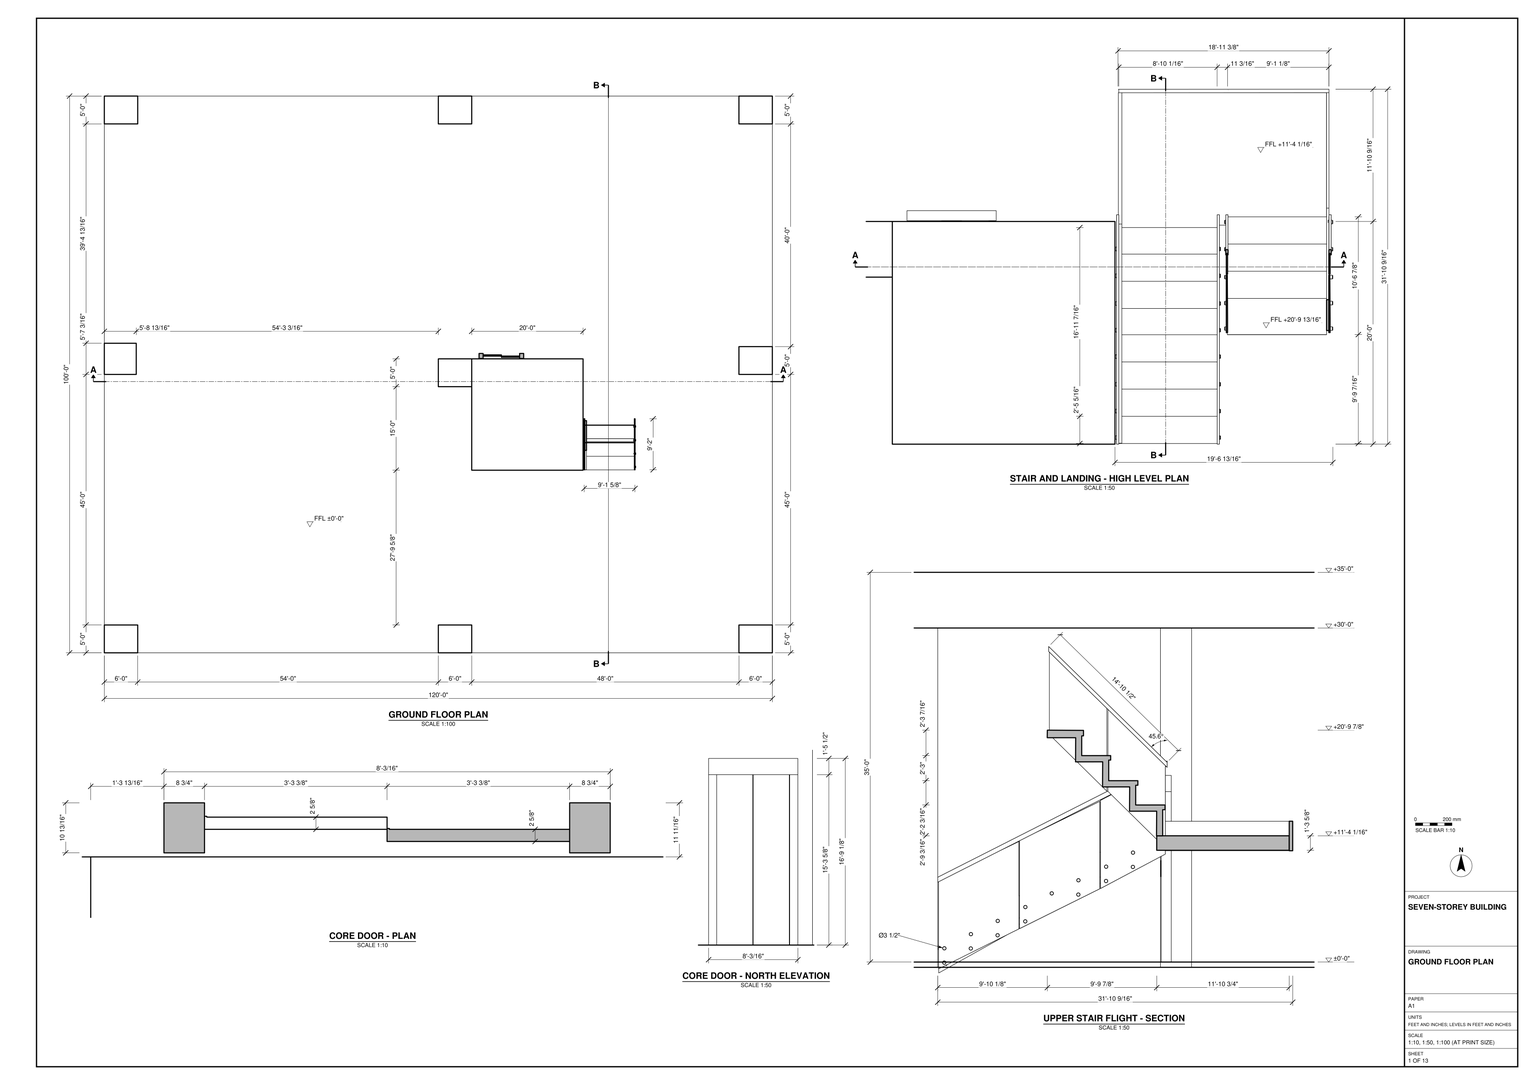
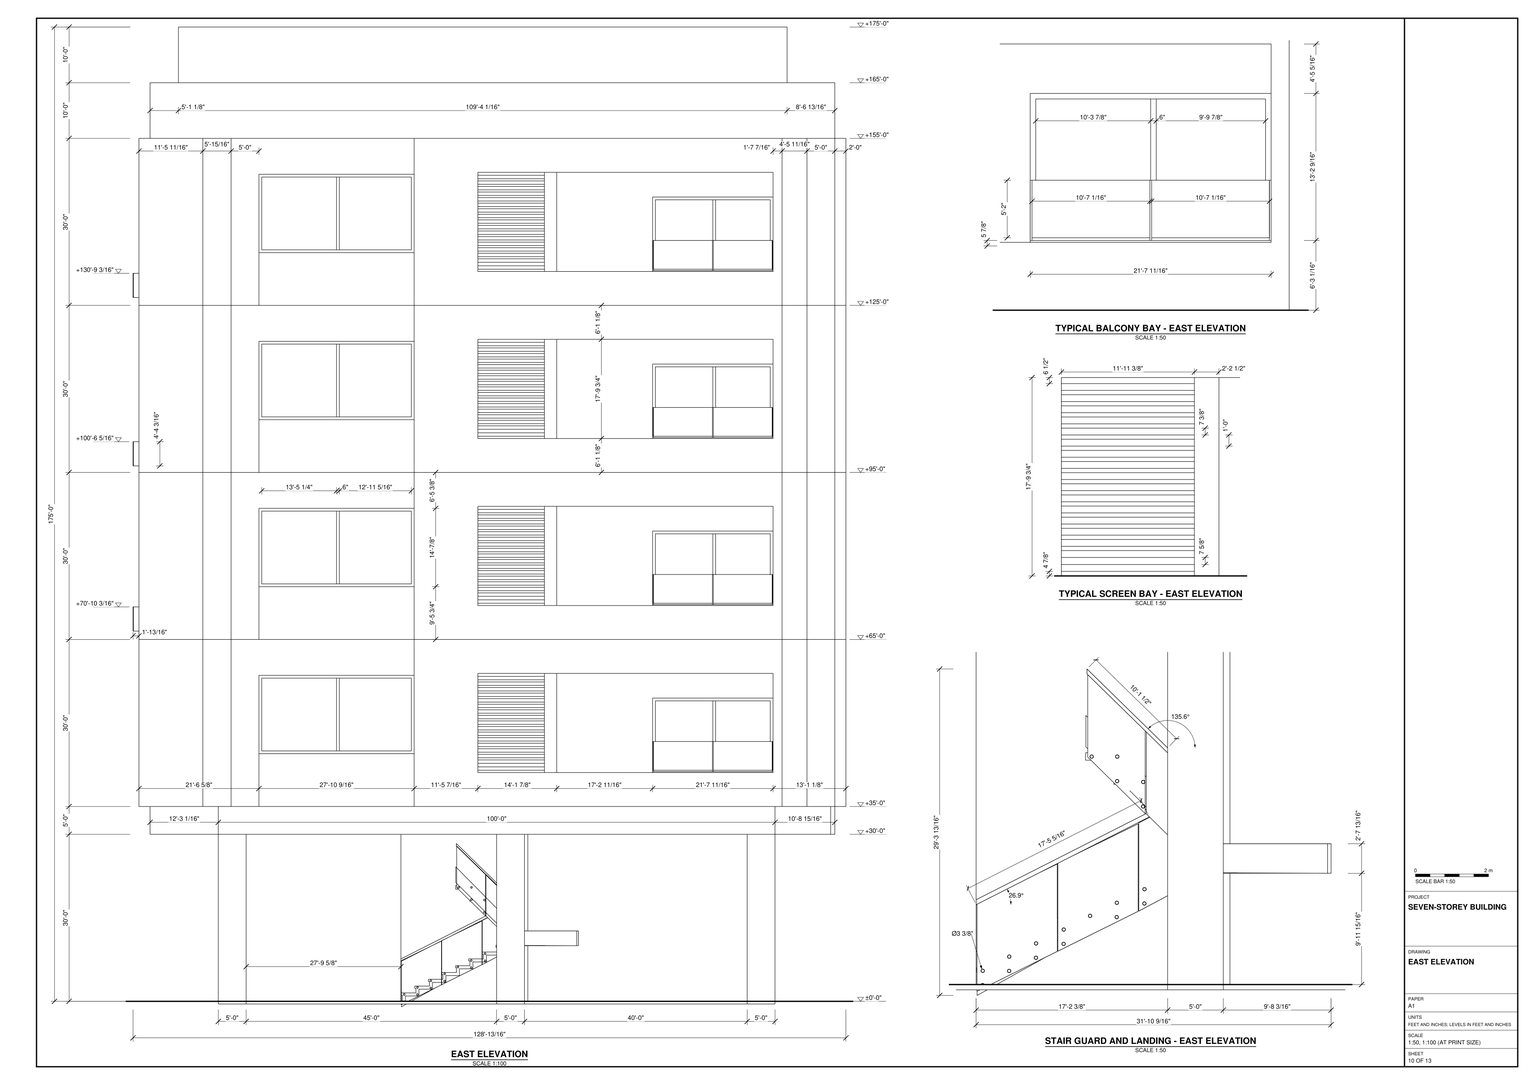
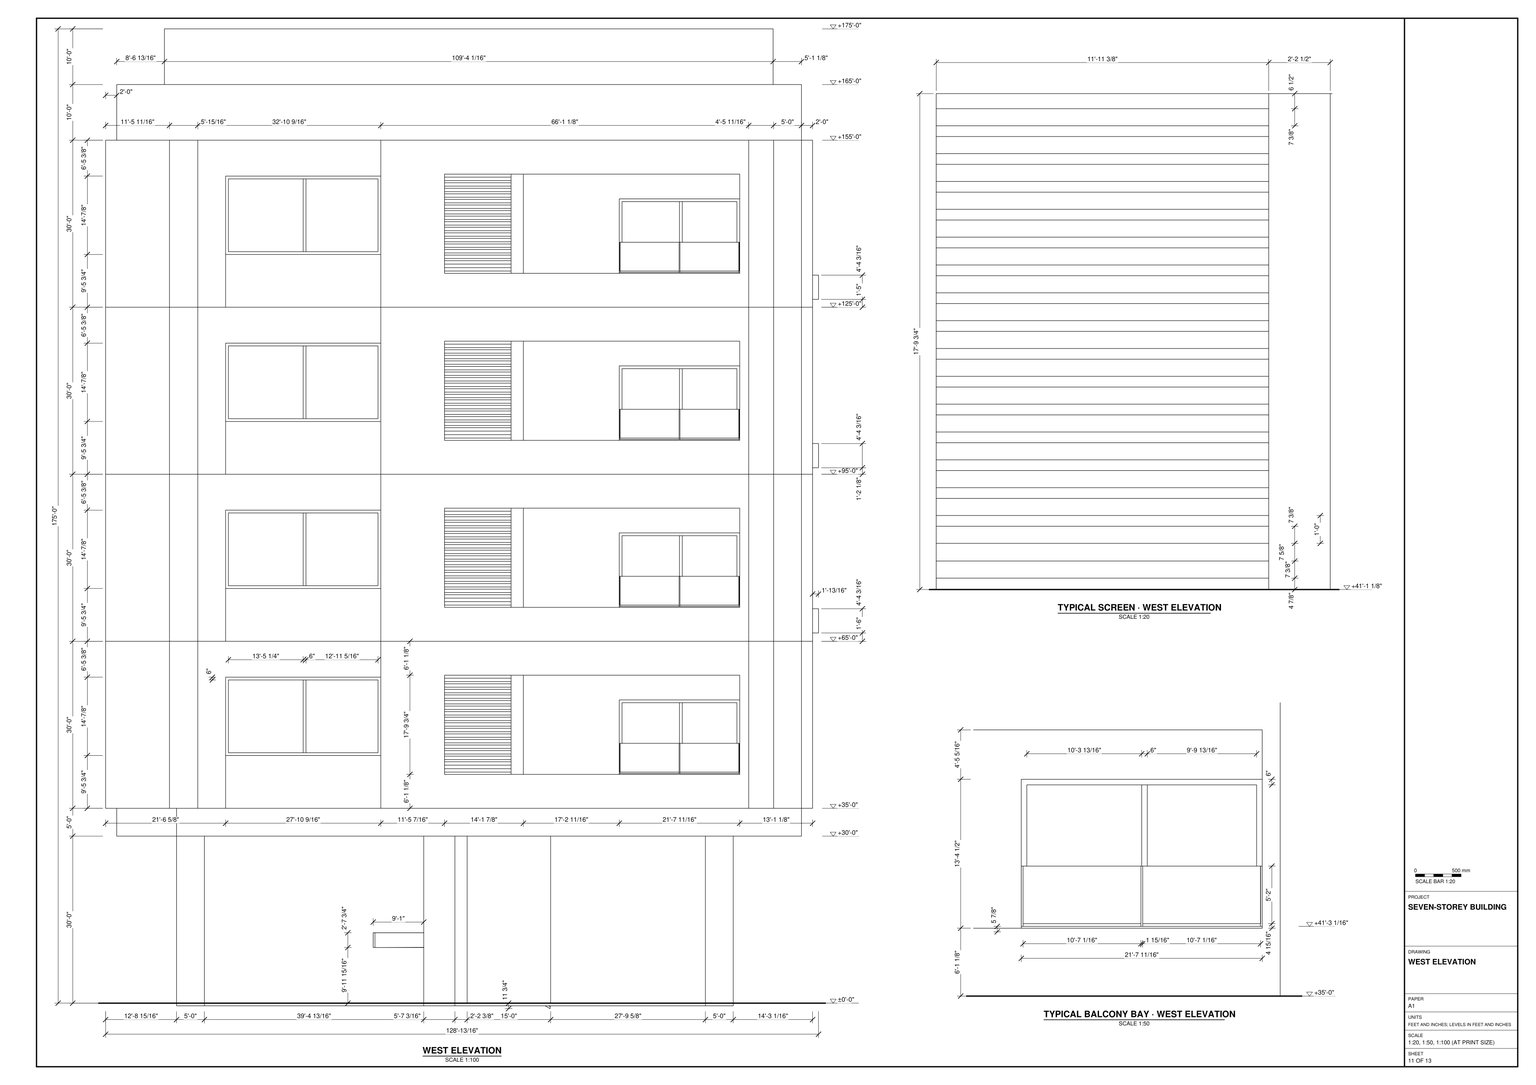
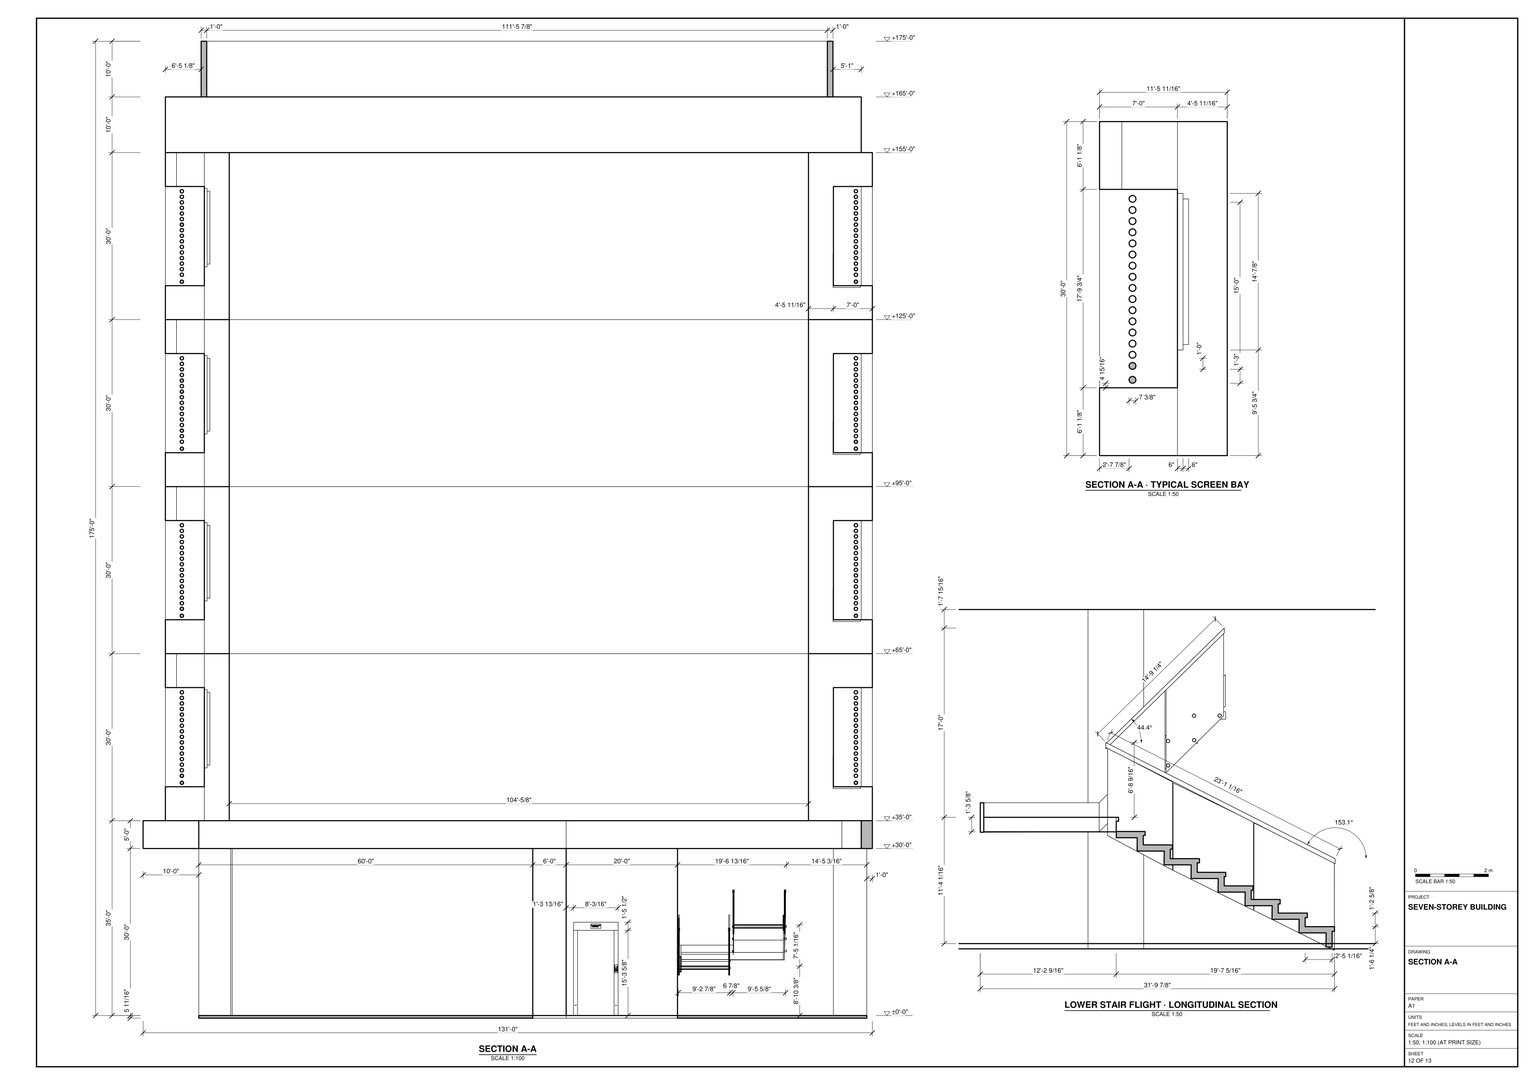
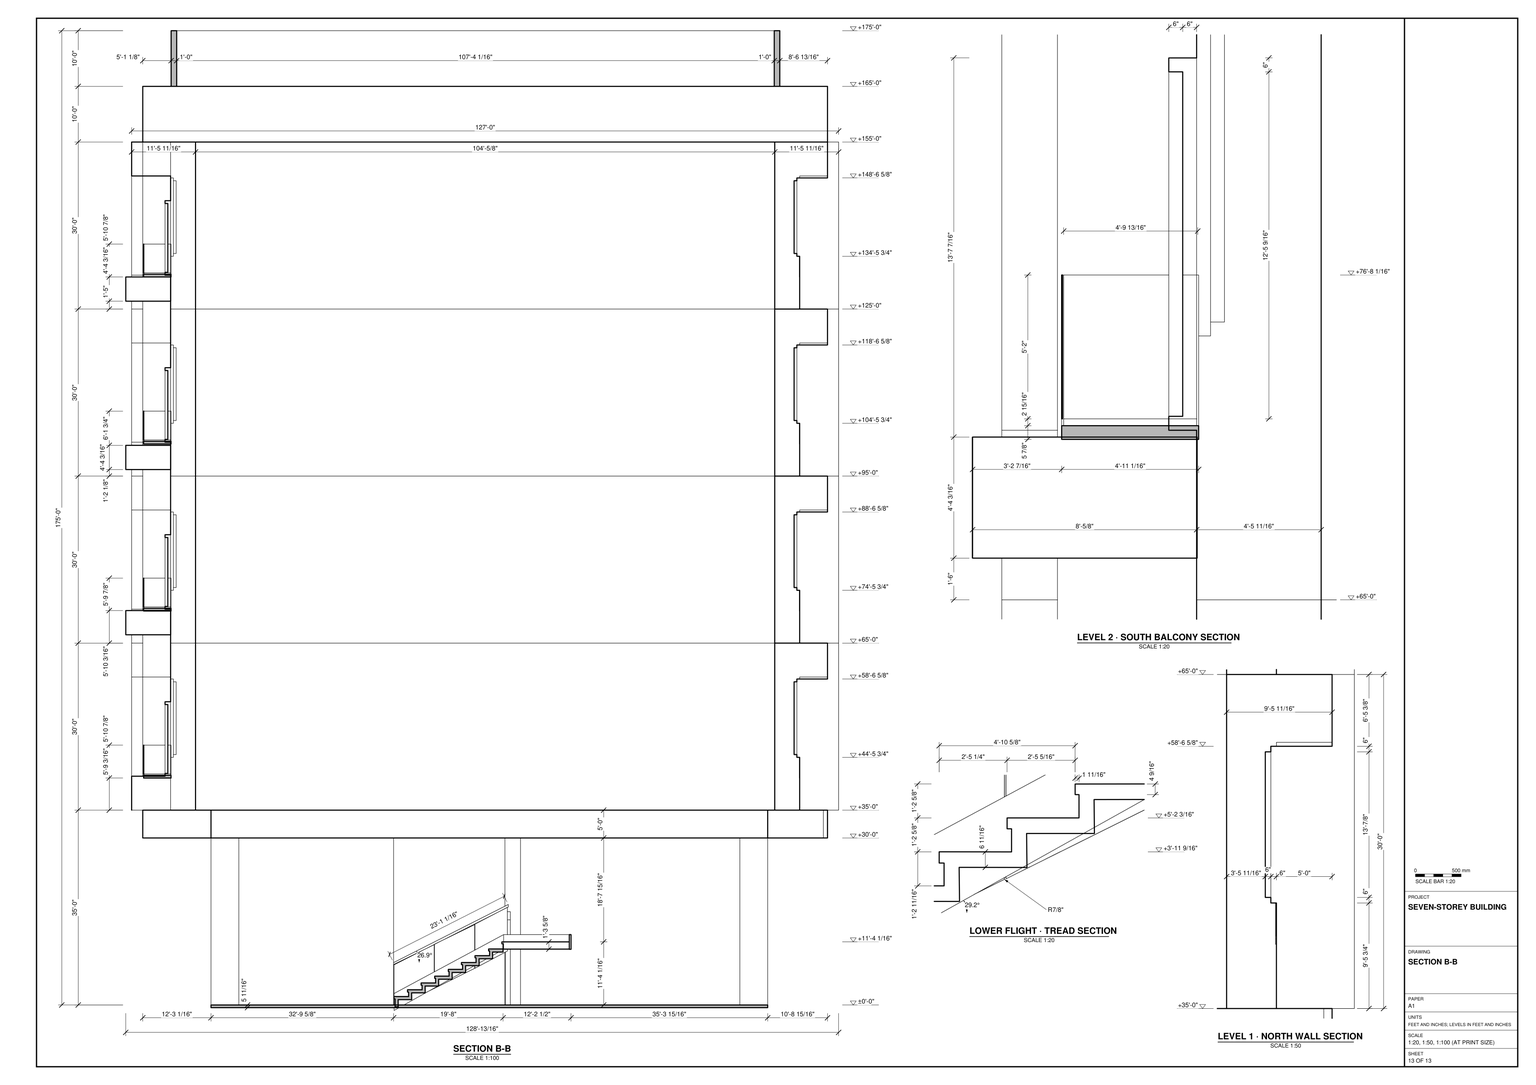
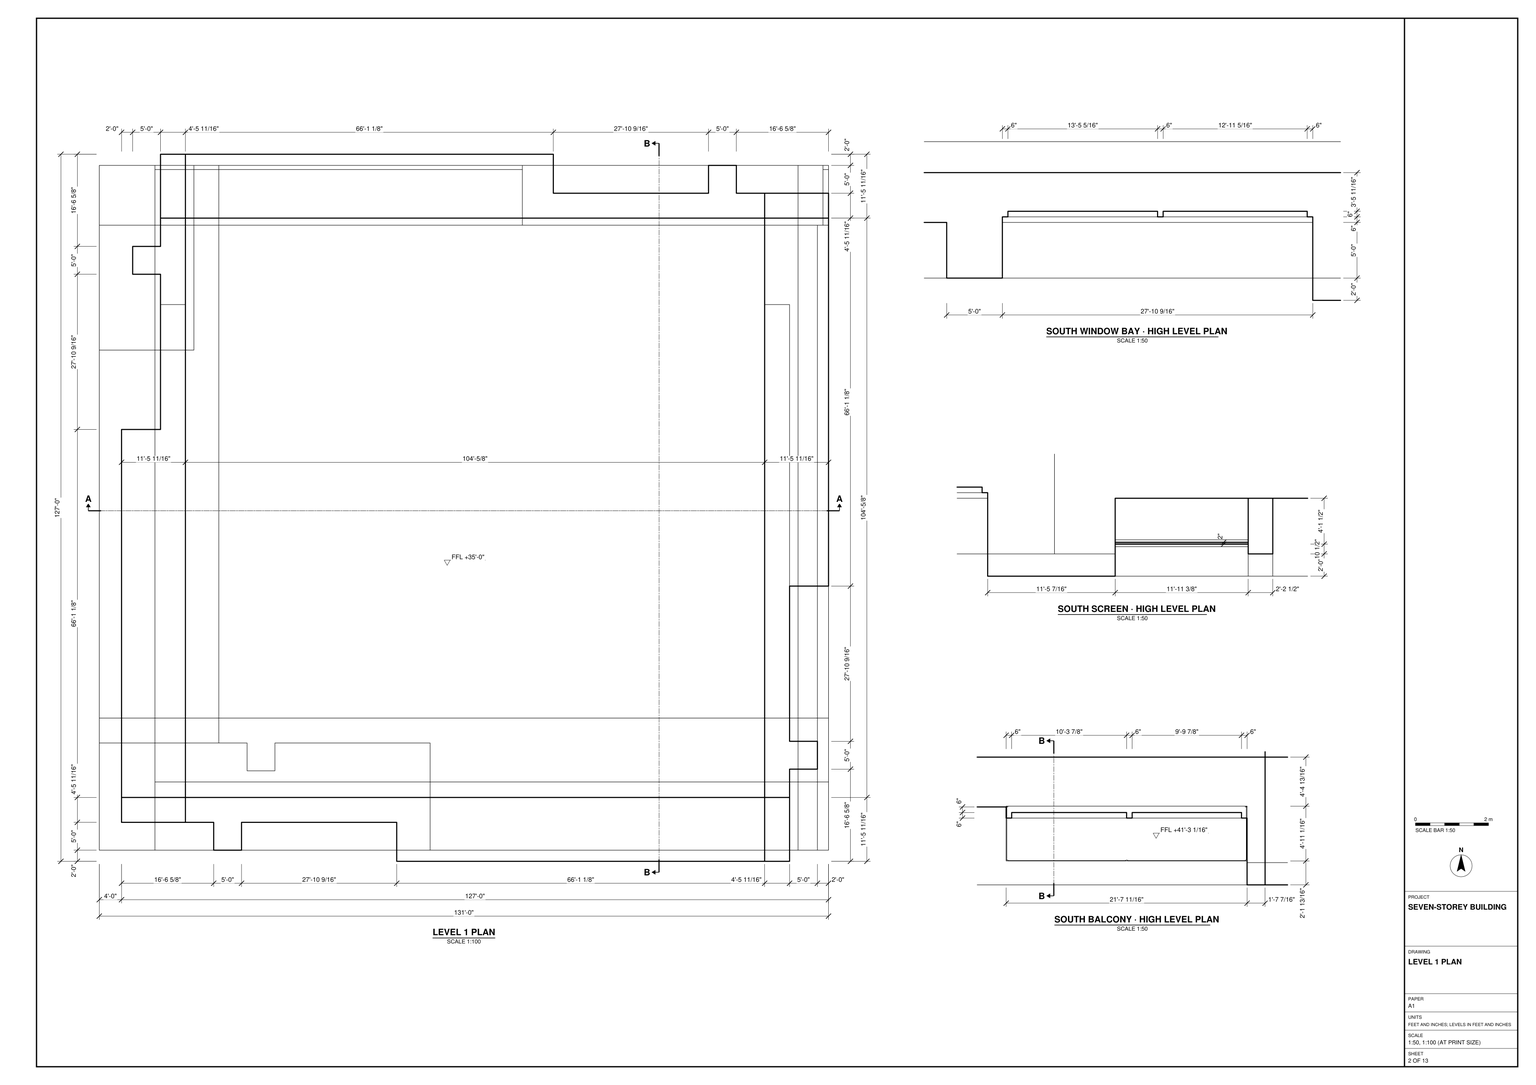
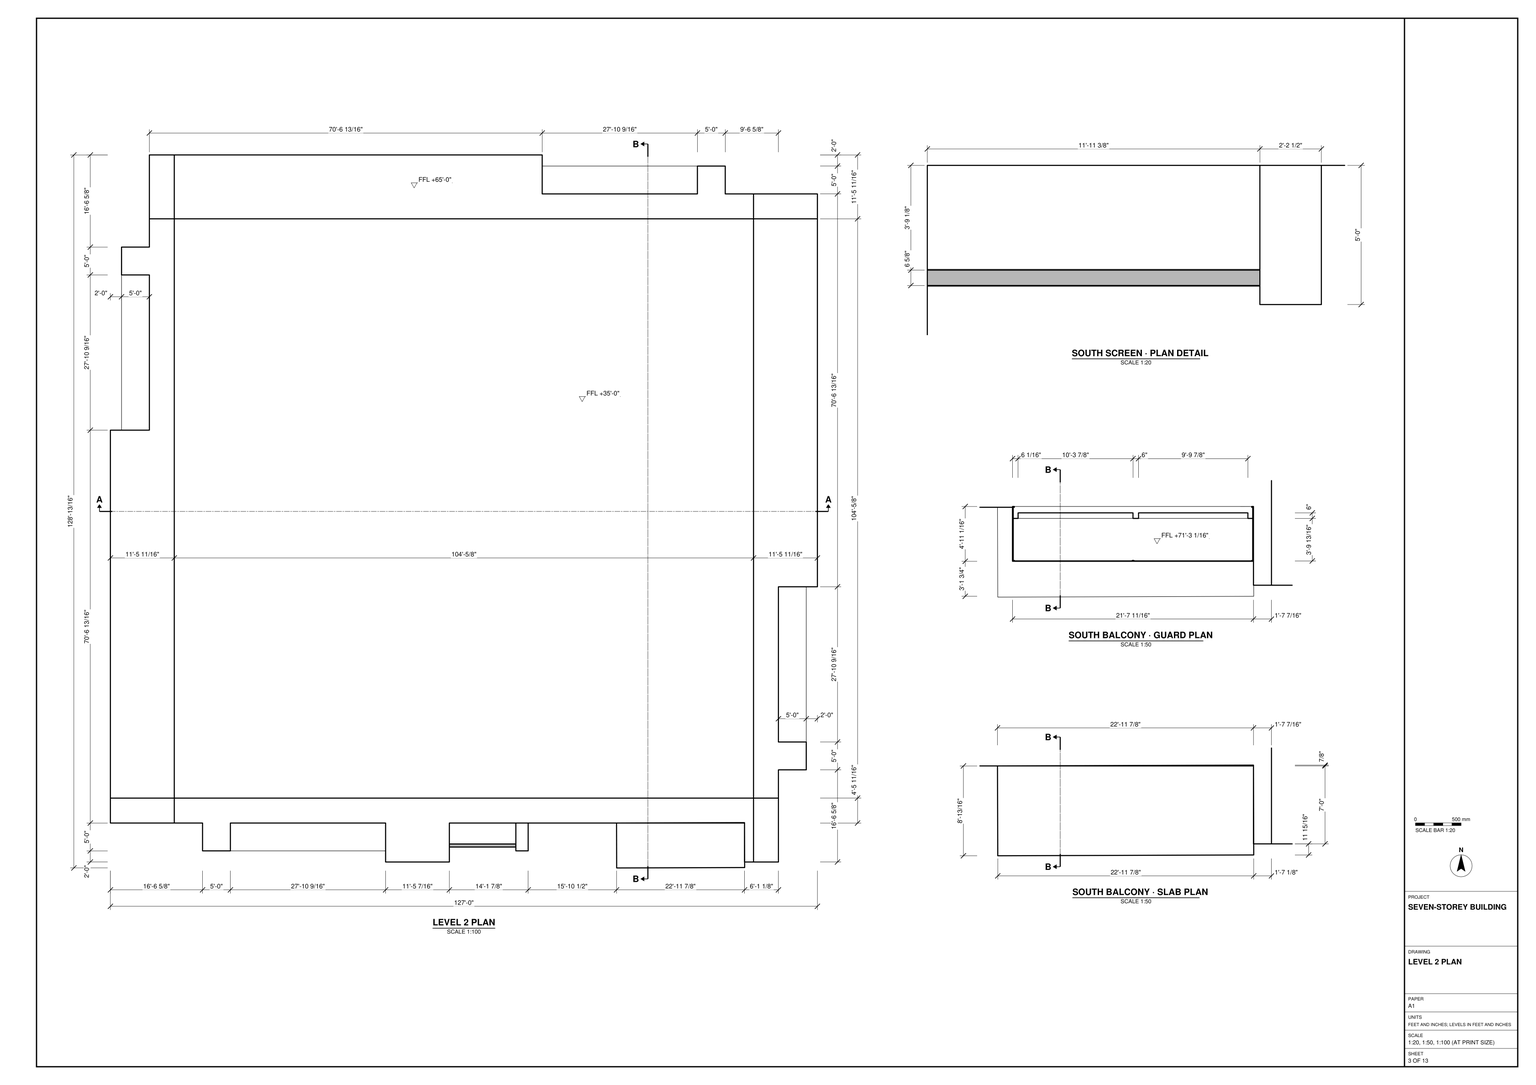
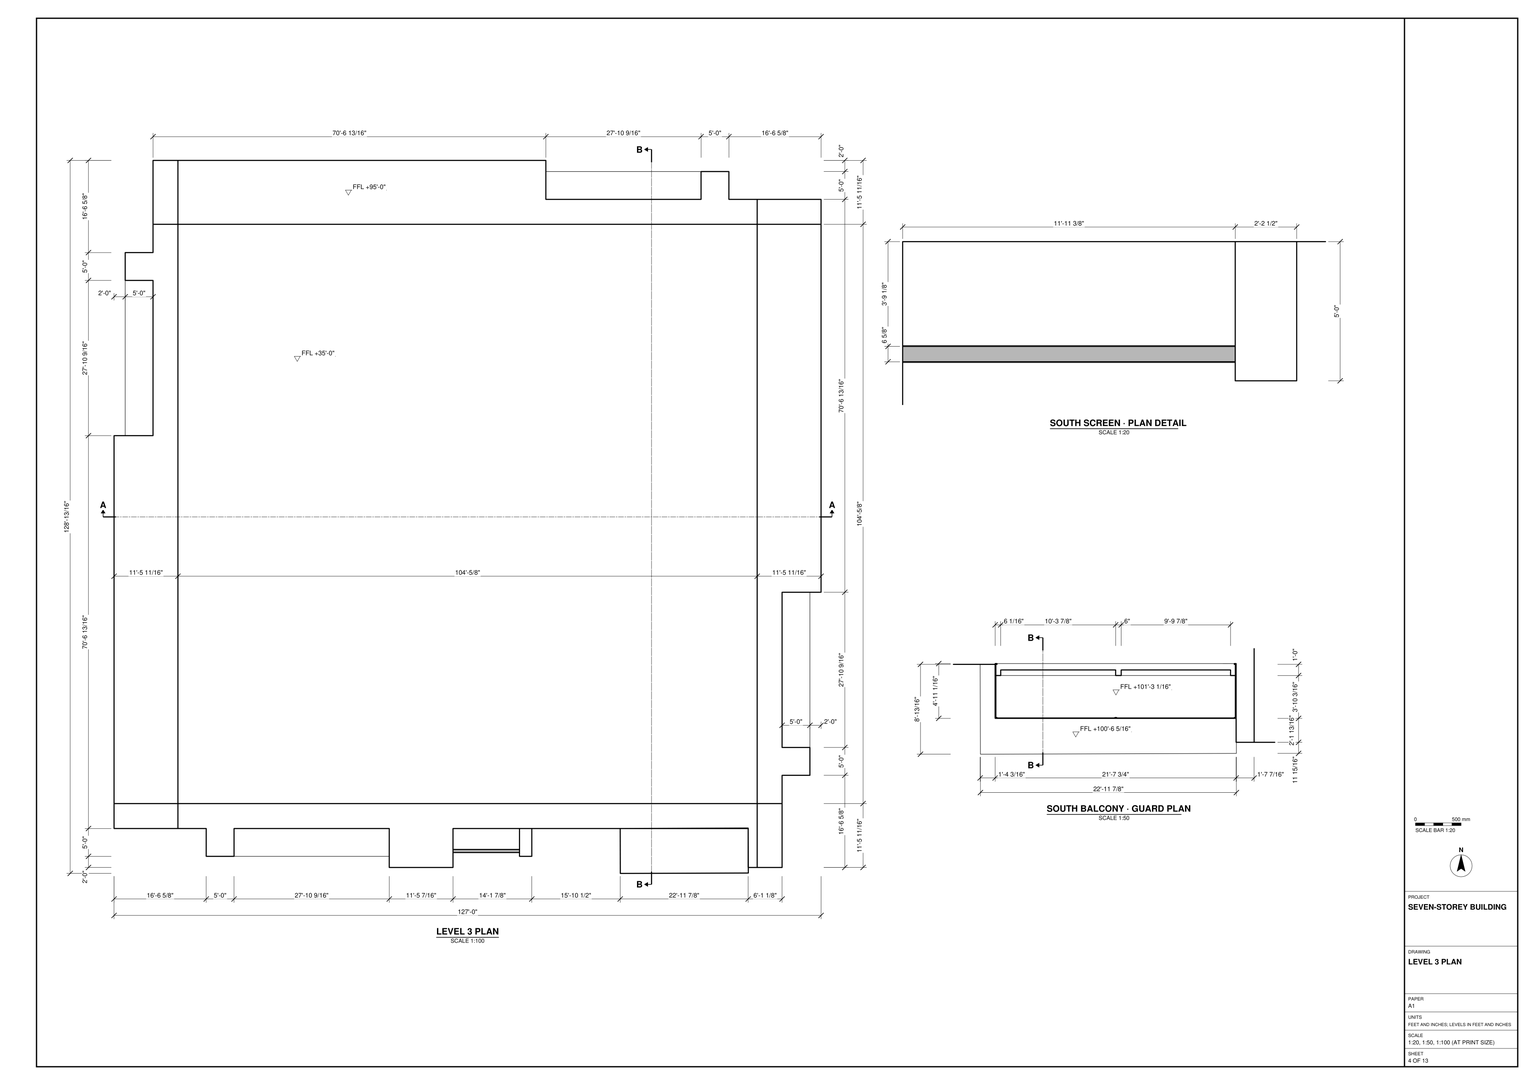
Build the seven-storey building in SketchUp from task_files/diagram_01.pdf. Work in feet and inches. The overall extents are 131'-0" along X, 128'-13/16" along Y and 175'-11 3/4" in height. Set the levels at ±0'-0", +35'-0", +65'-0", +95'-0", +125'-0", +155'-0" and +165'-0".

Lay out the rectangular ground-floor columns from the plan, keeping the space between them open except for the lift core and stair assembly. Use the enlarged details to model the core doorway, turning stair flights, landings and guards. Extend the slab over the columns to match the overhangs in elevation. Above it, model the floor slabs, walls at their drawn thicknesses, and door and window openings. On the east and west faces, align the paired window bays, horizontal screens and recessed balcony bays across the four repeating tiers. Include the balcony guards and finish the roof with the stepped profile shown in elevation.

Keep walls, slabs and roof elements in separate groups or components. Do the same for each furniture or joinery piece shown, and use components for repeated parts. Any decor or loose items shown may use suitable library components. Save one SketchUp model as output_files/seven_storey_building_with_open_column_supported_base.skp.

# SketchUp Ruby script. Lengths in inches.
U = 1.inch
M = Sketchup.active_model
def pt(a) = Geom::Point3d.new(a.map { |v| v * U })
def face(e, loops, mat)
  f = e.add_face(loops[0].map { |a| pt(a) })
  loops[1..].each { |l| e.add_face(l.map { |a| pt(a) }).erase! }
  f.material = f.back_material = mat if mat
  f
end
# faces: each face lists its corners as indices into pts; further lists are holes
def faces(e, pts, list, mat = nil) = list.each { |f| face(e, (f[0].is_a?(Array) ? f : [f]).map { |l| l.map { |i| pts[i] } }, mat) }
# xy, xz, yz: faces in a plane at the given z, y or x. An outline is a flat list of corners, or four numbers for a rectangle; further outlines are holes
def ring(l) = l.size == 4 ? [[l[0], l[1]], [l[2], l[1]], [l[2], l[3]], [l[0], l[3]]] : l.each_slice(2).to_a
def flat(e, list, mat, &to3) = list.each { |f| face(e, (f[0].is_a?(Array) ? f : [f]).map { |l| ring(l).map { |u, v| to3.(u, v) } }, mat) }
def xy(e, z, list, mat = nil) = flat(e, list, mat) { |x, y| [x, y, z] }
def xz(e, y, list, mat = nil) = flat(e, list, mat) { |x, z| [x, y, z] }
def yz(e, x, list, mat = nil) = flat(e, list, mat) { |y, z| [x, y, z] }
def lines(e, pts, list) = list.each { |a, b| e.add_line(pt(pts[a]), pt(pts[b])) }
# prism: a flat outline (further loops are holes) pulled along v
def prism(e, loops, v, mat = nil)
  f = face(e, loops, mat); d = Geom::Vector3d.new(v.map { |x| x * U })
  f.pushpull(f.normal.samedirection?(d) ? d.length : -d.length)
end
def box(e, o, s, mat = nil) = prism(e, [[o, [o[0] + s[0], o[1], o[2]], [o[0] + s[0], o[1] + s[1], o[2]], [o[0], o[1] + s[1], o[2]]]], [0, 0, s[2]], mat)
def at(x, y, z, deg = 0) = Geom::Transformation.translation(pt([x, y, z])) * Geom::Transformation.rotation(ORIGIN, Z_AXIS, deg.degrees)
def axes(o, x, y, z) = Geom::Transformation.new([*x, 0, *y, 0, *z, 0, *pt(o).to_a, 1])
def part(name) = M.definitions.add(name)
# library, detail: a bought-in or finely detailed component or shape, given as its bounding box
def library(name, o, s) = part(name).tap { |d| box(d.entities, o, s) }
def detail(e, o, s) = box(e.add_group.entities, o, s)
def put(e, d, t, mat = nil) = e.add_instance(d, t).tap { |i| i.material = mat if mat }
def group(e, t, mat = nil) = e.add_group.tap { |g| g.transformation = t; g.material = mat if mat }.entities
root = M.entities
M.materials.add("Matière par défaut71").color = [191, 191, 191]
M.materials.add("Porta Elevador").color = [142, 142, 142]
M.materials.add("[0042_Sienna]").color = [160, 82, 45]
M.materials.add("[0119_RosyBrown]").color = [234, 190, 174]
M.materials.add("[Color C07]").color = [216, 115, 55]
M.materials.add("wood").color = [204, 177, 156]
c1 = library("Porta Elevador",[0,0,0],[43.31,5.25,90.55])
c2 = part("Grouper\#4")
p = [[20.46,2457.84,0.01],[20.52,2457.51,0.05],[20.34,2457.64,0.03],[20.5625,2457.76,0],[20.5625,2492.17,0],[20.35,2492.15,0],
  [20.49,2492.39,0.01],[20.5625,2456.57,0.78],[20.375,2456.28,0.4375],[20.5,2456.62,0.48],[20.5625,2457.16,0.8],[20.5625,2456.91,0.71],
  [20.51,2457.05,0.41],[20.5625,2457.26,0.74],[20.55,2457.2,0.52],[20.5625,2456.66,295.05],[20.5625,2456.98,295.05],[20.53,2457.05,295.67],
  [20.5625,2457.18,295.05],[20.56,2457.1875,295.52],[20.5625,2457.37,295.24],[20.5625,2457.42,295.41],[20.5625,2457.26,295.54],[0,0.81,1592.54],
  [0,0.54,1592.43],[0.07,0.51,1592.89],[0.91,0,1593.5],[0.91,0.18,1593.65],[0.55,0.21,1593.59],[19.9375,0.21,1593.59],
  [19.58,0.18,1593.65],[19.58,0,1593.5]]
faces(c2.entities,p,[[0,1,2],[1,0,3],[4,5,6],[7,8,9],[10,11,12],[13,10,14],[15,16,17],[17,16,18],
  [19,18,20],[20,21,19],[21,22,19],[23,24,25],[26,27,28],[29,30,31]],"Matière par défaut71")
c3 = library("Grouper\#5",[0,0,0],[1856.49,2332.09,3252.59])
c4 = library("Grouper\#1",[0,0,0],[1815.27,2305.3,3203.6])
c5 = part("Grouper\#2")
xy(c5.entities,233.6875,[[0,0,849.2,24.21]],"wood")
xy(c5.entities,371.93,[[0,276.35,849.2,298.5]],"wood")
xy(c5.entities,510.17,[[0,552.91,849.2,572.72]],"wood")
xy(c5.entities,904.66,[[0,1456.88,849.2,1733.12]],"wood")
xy(c5.entities,967.36,[[0,1372.4,849.2,1669.76]],"wood")
xy(c5.entities,1063.14,[[0,1648.4,849.2,1668.78]],"wood")
xy(c5.entities,1178.47,[[0,2005.46,849.2,2218.53]],"wood")
xy(c5.entities,1201.38,[[0,1924.88,849.2,1944.27]],"wood")
xy(c5.entities,1233.61,[[2.35,2230.17,2.45,3564.97,32.5625,3564.97,32.47,2230.17]],"wood")
xy(c5.entities,1237.8,[[32.64,2219.03,1776.28,3565.13]],"wood")
xy(c5.entities,1241.18,[[0,1924.88,849.2,2218.53]],"wood")
xy(c5.entities,1345.2,[[32.64,2195,850.35,2219.03]],"wood")
xy(c5.entities,1383.22,[[931.04,2216.77,1777.375,2279.47]],"wood")
xy(c5.entities,1384.23,[[32.64,2195,850.35,2195,850.35,2219.03,1776.28,2219.03,1776.28,3565.13,32.64,3565.13]],"wood")
xy(c5.entities,1530.79,[[2.35,2230.17,32.47,2230.17,32.5625,3564.97,2.45,3564.97]],"wood")
xy(c5.entities,1531.46,[[1777.03,2392.14,1797.63,2392.14,1797.65,3565.96,1777.05,3565.96]],"wood")
xy(c5.entities,1647.78,[[931.04,2279.47,1777.375,2303.68]],"wood")
xy(c5.entities,1894.06,[[931.04,2005.18,1777.375,2027.33]],"wood")
xy(c5.entities,2148.05,[[931.04,1730.96,1777.375,1750.77]],"wood")
xz(c5.entities,0,[[0,233.6875,849.2,281.09]],"wood")
xz(c5.entities,3.19,[[3.34,0,32.44,342.3125]],"wood")
xz(c5.entities,24.21,[[0,74.42,849.2,233.6875]],"wood")
xz(c5.entities,276.35,[[0,371.93,849.2,418.34]],"wood")
xz(c5.entities,298.5,[[0,280.87,849.2,371.93]],"wood")
xz(c5.entities,552.91,[[0,510.17,849.2,555.59]],"wood")
xz(c5.entities,829.02,[[0,648.46,849.2,692.35]],"wood")
xz(c5.entities,847.08,[[0,555.16,849.2,648.37]],"wood")
xz(c5.entities,1109.05,[[1776.98,2508.5,1797.58,2825.33]],"wood")
xz(c5.entities,1121.37,[[0,692.3,849.2,786.42]],"wood")
xz(c5.entities,1372.4,[[0,925.2,849.2,967.36]],"wood")
xz(c5.entities,1395.66,[[0,829.45,849.2,925.1]],"wood")
xz(c5.entities,1456.6,[[931.04,2193.04,1777.375,2392.625]],"wood")
xz(c5.entities,1474.66,[[931.04,2392.72,1777.375,2447.9375]],"wood")
xz(c5.entities,1648.4,[[0,1063.14,849.2,1105.6]],"wood")
xz(c5.entities,1750.77,[[931.04,2148.05,1777.375,2193.47]],"wood")
xz(c5.entities,1924.88,[[0,1201.38,849.2,1241.18]],"wood")
xz(c5.entities,1944.27,[[0,1106.59,849.2,1201.38]],"wood")
xz(c5.entities,2005.18,[[931.04,1694.96,1777.375,1894.06]],"wood")
xz(c5.entities,2027.33,[[931.04,1894.06,1777.375,1940.47]],"wood")
xz(c5.entities,2195,[[32.64,1345.2,850.35,1384.23]],"wood")
xz(c5.entities,2218.53,[[0,1178.47,849.2,1241.18]],"wood")
xz(c5.entities,2219.03,[[32.64,1237.8,1776.28,1237.8,1776.28,1384.23,850.35,1384.23,850.35,1345.2,32.64,1345.2]],"wood")
xz(c5.entities,2230.17,[[2.35,1233.61,32.47,1530.79],[2.35,1233.61,32.47,1530.79]],"wood")
xz(c5.entities,2279.47,[[931.04,1383.22,1777.375,1647.78]],"wood")
xz(c5.entities,2303.68,[[931.04,1647.78,1777.375,1695.18]],"wood")
xz(c5.entities,2392.14,[[1777.03,1238.18,1777.03,1238.18,1797.63,1238.18,1797.63,1531.46,1777.03,1531.46,1777.03,1531.46],[1777.03,1238.18,1797.63,1531.46]],"wood")
xz(c5.entities,3564.97,[[2.45,1233.61,32.5625,1530.79]],"wood")
xz(c5.entities,3565.13,[[32.64,1237.8,1776.28,1384.23]],"wood")
xz(c5.entities,3565.96,[[1777.05,1233.02,1797.65,1531.46]],"wood")
yz(c5.entities,32.64,[[2219.03,1237.8,2219.03,1345.2,2195,1345.2,2195,1384.23,3565.13,1384.23,3565.13,1237.8]],"wood")
yz(c5.entities,850.35,[[2195,1345.2,2219.03,1384.23]],"wood")
yz(c5.entities,1776.28,[[2219.03,1237.8,3565.13,1384.23]],"wood")
p = [[2.35,2230.17,1233.61],[3.34,3.19,0],[3.34,3.19,342.3125],[2.35,2230.17,1530.79],[32.47,2230.17,1233.61],[32.44,3.19,0],
  [32.47,2230.17,1530.79],[32.44,3.19,342.3125],[2.99,3.51,44.61],[2.67,3.83,44.73],[2.96,3.79,44.54],[3.34,3.79,44.46],
  [3.34,3.48,44.57],[32.44,3.79,44.46],[32.44,3.48,44.57],[32.8,3.51,44.61],[32.82,3.79,44.54],[33.11,3.83,44.73],
  [2.96,4.11,44.59],[2.96,3.34,44.85],[2.67,3.51,44.95],[3.34,3.27,44.8125],[32.44,3.27,44.8125],[32.82,3.34,44.85],
  [33.11,3.51,44.95],[2.64,4.13,44.82],[2.5,3.8,45.04],[33.28,3.8,45.04],[2.43,4.15,45.18],[0,86.91,75.06],
  [849.2,86.91,75.06],[849.2,24.21,74.42],[0,24.21,74.42],[849.2,85.43,218.34],[0,85.43,218.34],[0,361.2,218.12],
  [849.2,361.2,218.12],[0,359.72,355.57],[849.2,359.72,355.57],[0,298.5,280.87],[0,0,281.09],[849.2,0,281.09],
  [849.2,298.5,280.87],[0,635.54,355.24],[849.2,635.54,355.24],[0,634.01,492.8],[849.2,634.01,492.8],[0,572.79,418.01],
  [0,276.35,418.34],[849.2,276.35,418.34],[849.2,572.79,418.01],[0,572.72,510.17],[849.2,572.72,510.17],[0,909.78,492.36],
  [849.2,909.78,492.36],[849.2,908.3,629.64],[0,908.3,629.64],[0,847.08,555.16],[0,552.91,555.59],[849.2,552.91,555.59],
  [849.2,847.08,555.16],[0,1184.07,629.59],[849.2,1184.07,629.59],[0,1182.59,766.48],[849.2,1182.59,766.48],[0,847.08,648.37],
  [849.2,847.08,648.37],[849.2,829.02,648.46],[0,829.02,648.46],[0,1121.37,692.3],[0,829.02,692.35],[849.2,829.02,692.35],
  [849.2,1121.37,692.3],[849.2,1458.36,766.8125],[0,1458.36,766.8125],[0,1456.88,904.66],[849.2,1456.88,904.66],[849.2,1121.37,786.42],
  [849.2,1105.63,786.5],[0,1105.64,786.5],[0,1121.37,786.42],[0,1105.64,829.12],[849.2,1105.63,829.12],[849.2,1395.66,829.45],
  [0,1395.66,829.45],[0,1733.12,904.66],[0,1730.58,1043.11],[849.2,1730.58,1043.11],[849.2,1733.12,904.66],[0,1372.4,925.2],
  [0,1395.66,925.1],[849.2,1395.66,925.1],[849.2,1372.4,925.2],[0,1668.78,1063.14],[0,1669.76,967.36],[849.2,1669.76,967.36],
  [849.2,1668.78,1063.14],[0,2006.98,1044.09],[849.2,2006.98,1044.09],[0,2005.46,1178.47],[849.2,2005.46,1178.47],[0,1944.27,1106.59],
  [0,1648.4,1105.6],[849.2,1648.4,1105.6],[849.2,1944.27,1106.59],[1797.65,3565.96,1233.02],[1797.63,2392.14,1238.18],[1777.03,2392.14,1238.18],
  [1777.05,3565.96,1233.02],[1777.05,3565.96,1531.46],[1777.03,2392.14,1531.46],[1797.65,3565.96,1531.46],[1797.63,2392.14,1531.46],[2.45,3564.97,1233.61],
  [1797.65,3565.96,1531.47],[2.45,3564.97,1530.79],[2.43,3600.13,1233.61],[1797.63,3601.12,1233.02],[1797.63,3601.11,1233.02],[1797.63,3601.09,1233.02],
  [1797.63,3601.0625,1233.02],[1797.63,3601.12,1529.03],[1797.63,3601.12,1531.47],[2.43,3600.13,1530.79],[32.5625,3564.97,1233.61],[32.5625,3564.97,1530.79],
  [1776.98,1109.05,2508.5],[1776.98,1109.05,2825.33],[1777.03,2392.14,1531.46],[1777.03,2392.14,1238.18],[1797.58,1109.05,2508.5],[1797.58,1109.05,2825.33],
  [1777.375,2216.77,1383.22],[1777.375,2218.25,1632.43],[931.04,2218.25,1632.43],[931.04,2216.77,1383.22],[1777.375,1942.48,1632.21],[931.04,1942.48,1632.21],
  [1777.375,1943.96,1877.7],[931.04,1943.96,1877.7],[931.04,2303.68,1695.18],[931.04,2005.18,1694.96],[1777.375,2005.18,1694.96],[1777.375,2303.68,1695.18],
  [1777.375,1668.14,1877.37],[931.04,1668.14,1877.37],[1777.375,1669.67,2130.68],[931.04,1669.67,2130.68],[1777.375,1730.89,1940.14],[1777.375,2027.33,1940.47],
  [931.04,2027.33,1940.47],[931.04,1730.89,1940.14],[1777.375,1730.96,2148.05],[931.04,1730.96,2148.05],[1777.375,1393.9,2130.24],[931.04,1393.9,2130.24],
  [1777.375,1395.38,2373.89],[931.04,1395.38,2373.89],[1777.375,1750.77,2193.47],[931.04,1750.77,2193.47],[931.04,1456.6,2193.04],[1777.375,1456.6,2193.04],
  [1777.375,1105.76,2373.84],[1777.375,1107.24,2450.15],[931.04,1107.24,2450.15],[931.04,1105.76,2373.84],[931.04,1456.6,2392.625],[931.04,1474.66,2392.72],
  [1777.375,1474.66,2392.72],[1777.375,1456.6,2392.625],[931.04,1474.66,2447.9375],[1777.375,1474.66,2447.9375]]
faces(c5.entities,p,[[0,1,2,3],[4,5,1,0],[5,4,6,7],[8,9,10],[11,12,8],[8,10,11],[12,11,13,14],[15,14,13],
  [13,16,15],[15,16,17],[18,10,9],[8,19,20],[8,12,21],[21,19,8],[21,12,14,22],[22,14,15],
  [15,23,22],[15,24,23],[20,9,8],[17,24,15],[9,25,18],[20,26,9],[17,27,24],[9,26,28],
  [28,25,9],[29,30,31,32],[33,30,29,34],[34,35,36,33],[35,37,38,36],[39,40,41,42],[2,7,6,3],[37,43,44,38],
  [43,45,46,44],[47,48,49,50],[51,47,50,52],[53,54,46,45],[55,54,53,56],[57,58,59,60],[56,61,62,55],[61,63,64,62],
  [65,66,67,68],[69,70,71,72],[73,64,63,74],[74,75,76,73],[77,78,79,80],[81,79,78,82],[82,83,84,81],[85,86,87,88],
  [89,90,91,92],[93,94,95,96],[86,97,98,87],[97,99,100,98],[101,102,103,104],[105,106,107,108],[109,108,107,110],[111,112,106,105],
  [113,105,111,114,115],[116,117,118,119,120,105,113],[121,122,114,111,105,120,119,118,117],[117,116,123,122,121],[0,3,115,113],[6,4,124,125],[123,116,113,115],[126,127,128,129],
  [106,130,126,129,107],[131,130,106,112],[132,133,134,135],[122,123,115,114],[131,112,110,128,127],[133,136,137,134],[136,138,139,137],[140,141,142,143],
  [138,144,145,139],[144,146,147,145],[148,149,150,151],[152,148,151,153],[146,154,155,147],[154,156,157,155],[158,159,160,161],[162,163,164,165],
  [156,162,165,157],[166,167,168,169],[170,164,163,171]],"wood")
c6 = part("Models (R_2) escalier quart tournant")
p = [[937.98,3563.27,1190.31],[937.97,3563.26,1190.42],[937.98,3563.37,1486.12],[937.98,3563.27,1486.34],[937.98,3598.92,1486.34],[937.98,3598.82,1486.12],
  [937.98,3563.49,1486.24],[937.98,3598.7,1486.24],[937.98,3563.37,1190.53],[937.98,3563.49,1190.41],[937.97,3563.4375,1486.34],[937.98,3563.47,1190.5],
  [937.98,3598.72,1486.14],[937.98,3598.92,1190.31],[937.98,3598.89,1190.33],[937.98,3598.82,1190.53],[937.98,3598.91,1190.33],[937.98,3598.86,1190.33],
  [937.98,3563.47,1486.14],[937.96,3598.8,1190.32],[78.3125,3589.58,1487.99],[78.33,3589.59,1488.11],[937.98,3598.72,1190.5],[937.98,3598.7,1190.41]]
lines(c6.entities,p,[[0,1],[2,3],[4,5],[3,6],[7,4],[0,8],[9,0],[3,10],[0,11],[4,12],[13,14],[15,16],
  [13,17],[3,18],[19,13],[20,21],[14,22],[17,23],[16,13]])
put(c6.entities,c2,at(917.42,1106.01,1190.31))
put(c6.entities,c3,at(-885.67,-8.88,-0.86))
put(c6.entities,c4,at(-867.875,-0.55,-0.86))
put(c6.entities,c5,at(-859.65,-2.2,-42.6875))
c7 = library("Group\#4",[0,0,0],[1524,1524,1440])
prism(root,[[[1139,96.8125,1516.98],[1414.89,97.68,1516.98],[1415.2,0.87,1516.98],[1139.3,0,1516.98]]],[0,0,52.19])
prism(root,[[[1139,96.8125,1154.11],[1414.89,97.68,1154.11],[1415.2,0.87,1154.11],[1139.3,0,1154.11]]],[0,0,52.19])
prism(root,[[[1139,96.8125,797.98],[1414.89,97.68,797.98],[1415.2,0.87,797.98],[1139.3,0,797.98]]],[0,0,52.19])
xy(root,-5.6875,[[[192,183.875,192,243.875,120,243.875,120,783.875,188.8125,783.875,188.8125,851.07,120,851.07,120,1323.875,192,1323.875,192,1383.875,840,1383.875,840,1323.875,912,1323.875,912,1383.875,1488,1383.875,1488,1323.875,1560,1323.875,1560,843.875,1488,843.875,1488,783.875,1560,783.875,1560,243.875,1488,243.875,1488,183.875,912,183.875,912,243.875,840,243.875,840,183.875],[912,577.47,1152,577.47,1152,817.47,840,817.47,840,757.47,912,757.47]]])
xy(root,0,[[[192,183.875,840,183.875,840,243.875,912,243.875,912,183.875,1488,183.875,1488,243.875,1560,243.875,1560,783.875,1488,783.875,1488,843.875,1560,843.875,1560,1323.875,1488,1323.875,1488,1383.875,912,1383.875,912,1323.875,840,1323.875,840,1383.875,192,1383.875,192,1323.875,120,1323.875,120,851.07,188.8125,851.07,188.8125,783.875,120,783.875,120,243.875,192,243.875],[912,577.47,912,757.47,840,757.47,840,817.47,1152,817.47,1152,577.47]],[840,183.875,912,243.875],[1488,183.875,1560,243.875],[912,577.47,1152,817.47],[840,757.47,912,817.47],
  [120,783.875,188.8125,851.07],[1488,783.875,1560,843.875],[840,1323.875,912,1383.875]])
xy(root,360,[[0,36.8125,120,243.875],[120,36.8125,192,183.875],[192,36.8125,840,183.875],[840,36.8125,912,183.875],[912,36.8125,1488,183.875],
  [1488,36.8125,1548,183.875],[1548,36.8125,1572,183.875],[120,183.875,192,243.875],[840,183.875,912,243.875],[1488,183.875,1548,243.875],
  [1548,183.875,1560,243.875],[1560,183.875,1572,243.875],[0,243.875,120,783.875],[1548,243.875,1572,783.875],[840,757.47,912,817.47],
  [0,783.875,120,851.07],[120,783.875,188.8125,851.07],[1488,783.875,1548,843.875],[1548,783.875,1560,843.875],[1560,783.875,1572,843.875],
  [1548,843.875,1572,1323.875],[0,851.07,120,1323.875],[0,1323.875,120,1383.875],[120,1323.875,192,1383.875],[840,1323.875,912,1383.875],
  [1488,1323.875,1548,1383.875],[1548,1323.875,1560,1383.875],[1560,1323.875,1572,1383.875],[0,1383.875,120,1512.8125],[120,1383.875,192,1503.875],
  [192,1383.875,840,1503.875],[840,1383.875,912,1503.875],[912,1383.875,1506.3125,1512.8125],[1506.3125,1383.875,1560,1512.8125],[1560,1383.875,1572,1503.875],
  [120,1503.875,192,1512.8125],[192,1503.875,840,1512.8125],[840,1503.875,912,1512.8125],[1560,1503.875,1572,1512.8125]])
xy(root,360,[[[192,183.875,840,183.875,840,243.875,912,243.875,912,183.875,1488,183.875,1488,243.875,1548,243.875,1548,783.875,1488,783.875,1488,843.875,1548,843.875,1548,1323.875,1488,1323.875,1488,1383.875,912,1383.875,912,1323.875,840,1323.875,840,1383.875,192,1383.875,192,1323.875,120,1323.875,120,851.07,188.8125,851.07,188.8125,783.875,120,783.875,120,243.875,192,243.875],[912,577.47,1152,817.47]],[912,577.47,1152,817.47]],"[Color C07]")
xy(root,420,[[0,36.8125,120,267.875],[120,36.8125,713.22,183.875],[713.22,36.8125,1506.3125,183.875],[1506.3125,36.8125,1548,183.875],[1548,36.8125,1572,183.875],
  [120,183.875,713.22,183.875,713.22,267.875,378.65,267.875,378.65,207.875,318.65,207.875,318.65,267.875,120,267.875],[713.22,183.875,1506.3125,183.875,1506.3125,321.5625,1548,321.5625,1548,1383.875,1506.3125,1383.875,1506.3125,321.5625,257.6875,321.5625,257.6875,267.875,318.65,267.875,318.65,207.875,378.65,207.875,378.65,267.875,713.22,267.875],[1506.3125,183.875,1548,321.5625],[1548,183.875,1572,321.5625],[0,267.875,120,321.5625],
  [120,267.875,257.6875,321.5625],[0,321.5625,120,1114.66],[120,321.5625,120,1114.66,204,1114.66,204,1383.875,257.6875,1383.875,257.6875,321.5625],[257.6875,321.5625,1506.3125,1383.875],[1548,321.5625,1572,1383.875],
  [0,1114.66,120,1383.875],[120,1114.66,204,1383.875],[0,1383.875,120,1512.8125],[120,1383.875,204,1503.875],[204,1383.875,257.6875,1503.875],
  [257.6875,1383.875,912,1503.875],[912,1383.875,1506.3125,1512.8125],[1506.3125,1383.875,1560,1512.8125],[1560,1383.875,1572,1503.875],[120,1503.875,204,1512.8125],
  [204,1503.875,257.6875,1512.8125],[257.6875,1503.875,912,1512.8125],[1560,1503.875,1572,1512.8125]])
xy(root,1860,[[48,36.8125,1548,1512.8125]])
xy(root,1980,[[[48,36.8125,1548,1512.8125],[125.14,97.94,1487.02,1410.01]],[[125.14,97.94,1487.02,1410.01],[137.14,109.94,1475.02,1398.01]]])
xy(root,1980,[[137.14,109.94,1475.02,1398.01]],"[0119_RosyBrown]")
xy(root,2100,[[[125.14,97.94,1487.02,1410.01],[137.14,109.94,1475.02,1398.01]]])
xz(root,36.8125,[[0,360,120,420],[120,360,1548,420],[1548,360,1572,420],[48,1860,1548,1980]])
xz(root,97.94,[[125.14,1980,1487.02,2100]],"[0119_RosyBrown]")
xz(root,109.94,[[137.14,1980,1475.02,2100]],"[0119_RosyBrown]")
xz(root,183.875,[[192,-5.6875,840,0],[912,-5.6875,1488,0],[120,0,192,360],[840,0,912,360],[1488,0,1560,360],
  [120,360,1548,420],[1548,360,1572,420]])
xz(root,243.875,[[120,-5.6875,192,360],[840,-5.6875,912,0],[1488,-5.6875,1560,0],[840,0,912,360],[1488,0,1560,360]])
xz(root,577.47,[[912,-5.6875,1152,0]])
xz(root,577.47,[[912,0,1152,360]],"[0042_Sienna]")
xz(root,757.47,[[840,-5.6875,912,0],[840,0,912,360]])
xz(root,783.875,[[120,-5.6875,188.8125,0],[1488,-5.6875,1560,0],[120,0,188.8125,360],[1488,0,1560,360]])
xz(root,817.47,[[840,-5.6875,912,0],[912,-5.6875,1152,0],[840,0,912,360]])
xz(root,817.47,[[912,0,1152,360]],"[Color C07]")
xz(root,843.875,[[1488,-5.6875,1560,0],[1488,0,1560,360]])
xz(root,851.07,[[120,-5.6875,188.8125,0],[120,0,188.8125,360]])
xz(root,1323.875,[[120,-5.6875,192,360],[840,-5.6875,912,0],[1488,-5.6875,1560,0],[840,0,912,360],[1488,0,1560,360]])
xz(root,1383.875,[[192,-5.6875,840,0],[912,-5.6875,1488,0],[120,0,192,360],[840,0,912,360],[1488,0,1560,360],
  [0,360,120,420],[120,360,912,420],[912,360,1506.3125,420],[1506.3125,360,1548,420],[1548,360,1572,420]])
xz(root,1398.01,[[137.14,1980,1475.02,2100]],"[0119_RosyBrown]")
xz(root,1410.01,[[125.14,1980,1487.02,2100]],"[0119_RosyBrown]")
xz(root,1503.875,[[120,360,912,420],[1560,360,1572,420]])
xz(root,1512.8125,[[0,360,120,420],[120,360,912,420],[912,360,1506.3125,420],[1506.3125,360,1560,420],[1560,360,1572,420],
  [48,1860,1548,1980]])
yz(root,0,[[36.8125,360,1383.875,420],[1383.875,360,1512.8125,420]])
yz(root,48,[[36.8125,1860,1512.8125,1980]])
yz(root,120,[[243.875,-5.6875,783.875,0],[851.07,-5.6875,1323.875,0],[183.875,0,243.875,360],[783.875,0,851.07,360],[1323.875,0,1383.875,360],
  [36.8125,360,183.875,420],[183.875,360,1383.875,420],[1383.875,360,1503.875,420],[1503.875,360,1512.8125,420]])
yz(root,125.14,[[97.94,1980,1410.01,2100]],"[0119_RosyBrown]")
yz(root,137.14,[[109.94,1980,1398.01,2100]],"[0119_RosyBrown]")
yz(root,188.8125,[[783.875,-5.6875,851.07,0],[783.875,0,851.07,360]])
yz(root,192,[[183.875,-5.6875,243.875,360],[1323.875,-5.6875,1383.875,360]])
yz(root,840,[[183.875,-5.6875,243.875,0],[757.47,-5.6875,817.47,0],[1323.875,-5.6875,1383.875,0],[183.875,0,243.875,360],[757.47,0,817.47,360],
  [1323.875,0,1383.875,360]])
yz(root,912,[[183.875,-5.6875,243.875,0],[577.47,-5.6875,757.47,0],[1323.875,-5.6875,1383.875,0],[183.875,0,243.875,360],[757.47,0,817.47,360],
  [1323.875,0,1383.875,360],[1383.875,360,1503.875,420],[1503.875,360,1512.8125,420]])
yz(root,912,[[577.47,0,757.47,360]],"[Color C07]")
yz(root,1152,[[577.47,-5.6875,817.47,0]])
yz(root,1152,[[577.47,0,817.47,360]],"[Color C07]")
yz(root,1475.02,[[109.94,1980,1398.01,2100]],"[0119_RosyBrown]")
yz(root,1487.02,[[97.94,1980,1410.01,2100]],"[0119_RosyBrown]")
yz(root,1488,[[183.875,-5.6875,243.875,0],[783.875,-5.6875,843.875,0],[1323.875,-5.6875,1383.875,360],[183.875,0,243.875,360],[783.875,0,843.875,360]])
yz(root,1506.3125,[[1383.875,360,1512.8125,420]])
yz(root,1548,[[36.8125,360,183.875,420],[183.875,360,1383.875,420],[36.8125,1860,1512.8125,1980]])
yz(root,1560,[[243.875,-5.6875,783.875,0],[843.875,-5.6875,1323.875,0],[183.875,0,243.875,360],[783.875,0,843.875,360],[1323.875,0,1383.875,360],
  [1503.875,360,1512.8125,420]])
yz(root,1572,[[36.8125,360,183.875,420],[183.875,360,1383.875,420],[1383.875,360,1503.875,420],[1503.875,360,1512.8125,420]])
put(root,c1,axes([927.78,817.47,0],[2.2213,0,0],[0,2.2213,0],[0,0,2.2213]))
put(root,c6,axes([1264.01,578.42,-7.2],[0.12647,0,0],[0,0.10604,0],[0,0,0.1068]))
g1 = group(root,at(48,12.8125,420))
xy(g1,0,[[1440,593.22,1440,1200,1386.3125,1200,1386.3125,1386.3125,1524,1386.3125,1524,593.22],[84,1200,84,1265.35,24,1265.35,24,1325.35,84,1325.35,84,1386.3125,137.6875,1386.3125,137.6875,1200],[84,1386.3125,137.6875,1524],[137.6875,1386.3125,137.6875,1524,930.78,1524,930.78,1440,1265.35,1440,1265.35,1500,1325.35,1500,1325.35,1440,1386.3125,1440,1386.3125,1386.3125]])
put(g1,c7,at(0,0,0))
